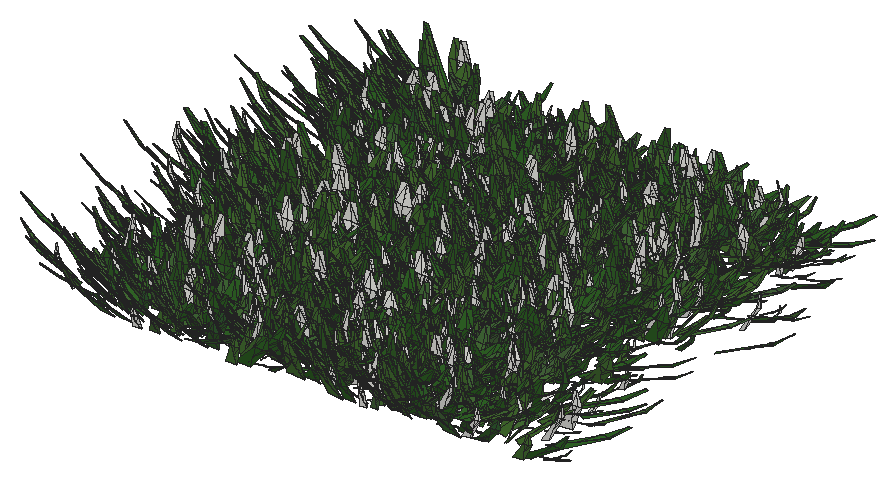
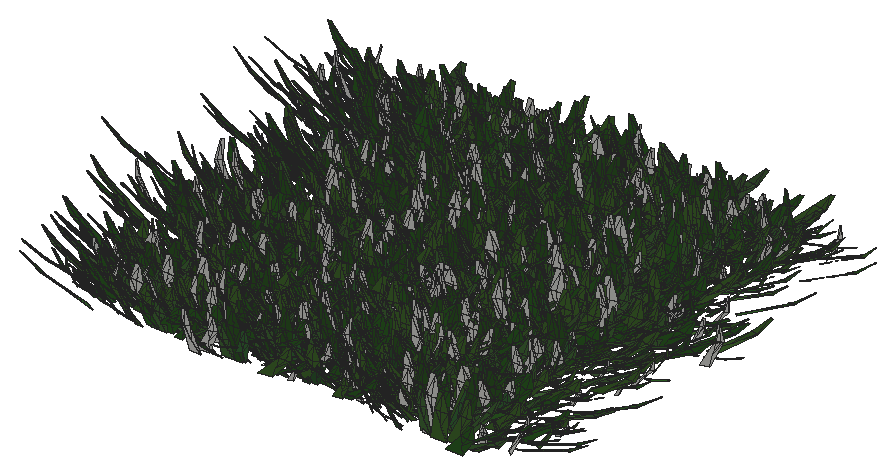
# SketchUp Ruby script. Lengths in inches.
U = 1.inch
M = Sketchup.active_model
def pt(a) = Geom::Point3d.new(a.map { |v| v * U })
def face(e, loops, mat)
  f = e.add_face(loops[0].map { |a| pt(a) })
  loops[1..].each { |l| e.add_face(l.map { |a| pt(a) }).erase! }
  f.material = f.back_material = mat if mat
  f
end
# faces: each face lists its corners as indices into pts; further lists are holes
def faces(e, pts, list, mat = nil) = list.each { |f| face(e, (f[0].is_a?(Array) ? f : [f]).map { |l| l.map { |i| pts[i] } }, mat) }
# xy, xz, yz: faces in a plane at the given z, y or x. An outline is a flat list of corners, or four numbers for a rectangle; further outlines are holes
def ring(l) = l.size == 4 ? [[l[0], l[1]], [l[2], l[1]], [l[2], l[3]], [l[0], l[3]]] : l.each_slice(2).to_a
def flat(e, list, mat, &to3) = list.each { |f| face(e, (f[0].is_a?(Array) ? f : [f]).map { |l| ring(l).map { |u, v| to3.(u, v) } }, mat) }
def xy(e, z, list, mat = nil) = flat(e, list, mat) { |x, y| [x, y, z] }
def xz(e, y, list, mat = nil) = flat(e, list, mat) { |x, z| [x, y, z] }
def yz(e, x, list, mat = nil) = flat(e, list, mat) { |y, z| [x, y, z] }
def lines(e, pts, list) = list.each { |a, b| e.add_line(pt(pts[a]), pt(pts[b])) }
# prism: a flat outline (further loops are holes) pulled along v
def prism(e, loops, v, mat = nil)
  f = face(e, loops, mat); d = Geom::Vector3d.new(v.map { |x| x * U })
  f.pushpull(f.normal.samedirection?(d) ? d.length : -d.length)
end
def box(e, o, s, mat = nil) = prism(e, [[o, [o[0] + s[0], o[1], o[2]], [o[0] + s[0], o[1] + s[1], o[2]], [o[0], o[1] + s[1], o[2]]]], [0, 0, s[2]], mat)
def at(x, y, z, deg = 0) = Geom::Transformation.translation(pt([x, y, z])) * Geom::Transformation.rotation(ORIGIN, Z_AXIS, deg.degrees)
def axes(o, x, y, z) = Geom::Transformation.new([*x, 0, *y, 0, *z, 0, *pt(o).to_a, 1])
def part(name) = M.definitions.add(name)
# library, detail: a bought-in or finely detailed component or shape, given as its bounding box
def library(name, o, s) = part(name).tap { |d| box(d.entities, o, s) }
def detail(e, o, s) = box(e.add_group.entities, o, s)
def put(e, d, t, mat = nil) = e.add_instance(d, t).tap { |i| i.material = mat if mat }
def group(e, t, mat = nil) = e.add_group.tap { |g| g.transformation = t; g.material = mat if mat }.entities
root = M.entities
M.materials.add("Material10").color = [48, 100, 38]
M.materials.add("Material3").color = [68, 110, 58]
M.materials.add("Material4").color = [48, 90, 38]
M.materials.add("Material5").color = [68, 110, 48]
M.materials.add("Material6").color = [48, 90, 48]
M.materials.add("Material7").color = [58, 110, 58]
M.materials.add("Material8").color = [58, 90, 38]
M.materials.add("Material9").color = [68, 100, 58]
c1 = part("grass00")
p = [[-0.6875,0.15,0],[-0.56,0.08,5.52],[-0.04,0.03,2.76],[0.48,-0.02,0],[0.35,-0.02,5.52],[-0.1,-0.14,5.52],
  [-0.12,0.65,8.37],[-0.42,0.65,8.37]]
faces(c1.entities,p,[[0,1,2,3],[3,2,4],[1,5,2],[5,4,2],[1,6,5],[4,5,6],[7,6,1]])
c2 = part("Group16\#1")
put(c2.entities,c1,axes([1.44,-0.61,-0.01],[0.05352,0.12609,0],[-0.10704,0.04543,0.07239],[0.06664,-0.02828,0.11628]),"Material6")
put(c2.entities,c1,axes([0.76,-0.15,-0.01],[0.04676,0.24062,0],[-0.23162,0.04501,0.06642],[0.0652,-0.01267,0.23595]),"Material3")
put(c2.entities,c1,axes([0.79,0.01,-0.01],[-0.00606,0.34651,0],[-0.34381,-0.00602,0.0432],[0.04319,0.00076,0.34386]))
put(c2.entities,c1,axes([1,0.23,-0.01],[-0.07192,0.31144,0],[-0.28722,-0.06632,0.1236],[0.12043,0.02781,0.29478]),"Material5")
put(c2.entities,c1,axes([1.66,0.77,-0.01],[-0.13828,0.29651,0],[-0.21551,-0.1005,0.22471],[0.20365,0.09498,0.23779]),"Material10")
put(c2.entities,c1,axes([0.6875,0.52,-0.01],[-0.18126,0.24051,0],[-0.22746,-0.17142,0.09788],[0.07817,0.05891,0.28481]),"Material5")
put(c2.entities,c1,axes([0.68,0.78,-0.01],[-0.215,0.18688,0],[-0.12385,-0.14248,0.21334],[0.13995,0.16101,0.18878]),"Material3")
put(c2.entities,c1,axes([0.56,1,-0.01],[-0.13756,0.07624,0],[-0.06159,-0.11112,0.0927],[0.04494,0.08108,0.12705]),"Material5")
put(c2.entities,c1,axes([0.2,0.64,-0.01],[-0.23729,0.07254,0],[-0.05711,-0.18681,0.153],[0.04473,0.14632,0.19535]),"Material10")
put(c2.entities,c1,axes([0.0625,0.72,-0.01],[-0.28874,0.02525,0],[-0.02179,-0.24916,0.14647],[0.01276,0.14591,0.25012]),"Material3")
put(c2.entities,c1,axes([-0.08,0.62,-0.01],[-0.34089,-0.04187,0],[0.03255,-0.26504,0.216],[-0.02633,0.21439,0.26703]),"Material10")
put(c2.entities,c1,axes([-0.34,0.98,-0.01],[-0.14314,-0.0493,0],[0.04397,-0.12769,0.06843],[-0.02228,0.0647,0.13505]),"Material10")
put(c2.entities,c1,axes([-0.87,1.45,-0.01],[-0.23488,-0.14114,0],[0.13761,-0.22901,0.06087],[-0.03135,0.05217,0.26717]))
put(c2.entities,c1,axes([-0.72,0.77,-0.01],[-0.14208,-0.13251,0],[0.07209,-0.0773,0.16301],[-0.11118,0.11922,0.1057]),"Material10")
put(c2.entities,c1,axes([-0.62,0.43,-0.01],[-0.14845,-0.21203,0],[0.18654,-0.13061,0.12304],[-0.10079,0.07057,0.22772]),"Material3")
put(c2.entities,c1,axes([-0.68,0.29,-0.01],[-0.13639,-0.32136,0],[0.31723,-0.13464,0.05579],[-0.05136,0.0218,0.34462]),"Material4")
put(c2.entities,c1,axes([-0.64,0.125,-0.01],[-0.0458,-0.23569,0],[0.22124,-0.043,0.08276],[-0.08124,0.01579,0.22538]),"Material7")
put(c2.entities,c1,axes([-1.6,-0.03,-0.01],[0.00576,-0.32897,0],[0.27526,0.00482,0.18018],[-0.18015,-0.00315,0.2753]),"Material5")
put(c2.entities,c1,axes([-1.36,-0.31,-0.01],[0.05718,-0.24765,0],[0.18172,0.04196,0.17267],[-0.16825,-0.03885,0.1865]),"Material10")
put(c2.entities,c1,axes([-1.54,-0.72,-0.01],[0.06537,-0.14017,0],[0.13555,0.06321,0.03939],[-0.0357,-0.01665,0.14956]))
put(c2.entities,c1,axes([-1.19,-0.9,-0.01],[0.09597,-0.12735,0],[0.11214,0.08451,0.07557],[-0.06035,-0.04548,0.14042]),"Material9")
put(c2.entities,c1,axes([-0.47,-0.54,-0.01],[0.11588,-0.10072,0],[0.0618,0.0711,0.12124],[-0.07953,-0.0915,0.0942]))
put(c2.entities,c1,axes([-0.47,-0.84,-0.01],[0.11927,-0.0661,0],[0.06603,0.11913,0.00646],[-0.00313,-0.00565,0.13621]),"Material5")
put(c2.entities,c1,axes([-0.38,-1.24,-0.01],[0.28037,-0.08571,0],[0.0618,0.20215,0.20315],[-0.05939,-0.19428,0.21139]),"Material9")
put(c2.entities,c1,axes([-0.06,-0.66,-0.01],[0.22719,-0.01987,0],[0.01247,0.14255,0.17758],[-0.01547,-0.17691,0.1431]),"Material8")
put(c2.entities,c1,axes([0.11,-0.89,-0.01],[0.14882,0.01828,0],[-0.01058,0.08611,0.12229],[0.01491,-0.12138,0.08676]),"Material6")
put(c2.entities,c1,axes([0.25,-0.72,-0.01],[0.20481,0.07053,0],[-0.06206,0.18022,0.10291],[0.03351,-0.0973,0.1906]),"Material6")
put(c2.entities,c1,axes([0.85,-1.42,-0.01],[0.16481,0.09904,0],[-0.09472,0.15762,0.05616],[0.02893,-0.04814,0.18389]),"Material5")
put(c2.entities,c1,axes([1.01,-1.09,-0.01],[0.21858,0.20385,0],[-0.17495,0.1876,0.15339],[0.10462,-0.11218,0.25652]),"Material10")
put(c2.entities,c1,axes([1.01,-0.71,-0.01],[0.08733,0.12473,0],[-0.06445,0.04512,0.13037],[0.1068,-0.07477,0.07867]),"Material6")
c3 = part("Group15\#1")
put(c3.entities,c2,at(0,0,0))
c4 = part("3darcstudiotree_grass00\#1")
put(c4.entities,c3,at(0,0,0))
put(root,c4,axes([257.86,22.3125,7.6],[3.70549,0.72715,0],[-2.49617,0.79502,-0.02005],[-0.09119,0.02904,1.86077]))
put(root,c4,axes([260.11,41.54,7.6],[0.01218,-1.00906,0],[4.98185,0.00376,-0.03692],[0.18714,0.00014,1.57831]))
put(root,c4,axes([260.48,26.33,7.6],[-1.42025,-0.83489,0],[4.16242,-0.44255,-0.01791],[0.11075,-0.01178,1.89984]))
put(root,c4,axes([260.59,11.3125,7.6],[0.28027,-0.96199,0],[3.64955,0.06646,-0.00937],[0.0792,0.00144,1.93766]))
put(root,c4,axes([260.47,8.13,7.6],[-3.43805,0.34453,0],[-1.648,-1.02783,-0.04281],[-0.10438,-0.0651,1.81418]))
put(root,c4,axes([260.35,37.81,7.6],[3.40925,-0.75567,0],[3.0298,0.85432,-0.03392],[0.10448,0.02946,1.32537]))
put(root,c4,axes([261.56,15.87,7.6],[-4.27926,0.10077,0],[-0.4125,-1.0948,-0.0202],[-0.01348,-0.03577,1.95637]))
put(root,c4,axes([260.31,4.91,7.6],[3.9837,-0.03206,0],[0.11597,0.90077,-0.04101],[0.00803,0.06239,1.37186]))
put(root,c4,axes([260.38,43.39,7.6],[0.14781,1.06815,0],[-4.11052,0.03555,-0.02489],[-0.18669,0.00161,1.9295]))
put(root,c4,axes([261,40.27,7.6],[-2.74206,0.64257,0],[-3.29567,-0.87899,-0.02311],[-0.07278,-0.01941,1.38694]))
put(root,c4,axes([262.26,35.6,7.6],[-4.52462,0.16915,0],[-0.75823,-1.26762,-0.06496],[-0.05656,-0.09455,1.88637]))
put(root,c4,axes([261.375,23.73,7.6],[-1.87065,0.77621,0],[-4.34622,-0.65464,-0.04504],[-0.23728,-0.03574,1.9506]))
put(root,c4,axes([261.58,30.06,7.6],[4.16044,-0.73269,0],[2.40364,0.85303,-0.03692],[0.14968,0.05312,1.83631]))
put(root,c4,axes([261.44,6.63,7.6],[3.59915,0.14594,0],[-0.59052,0.91023,-0.01255],[-0.01426,0.02198,1.63564]))
put(root,c4,axes([262.1,34.35,7.6],[-2.60039,0.90097,0],[-2.99223,-0.53976,-0.00844],[-0.04191,-0.00756,1.41311]))
put(root,c4,axes([261.36,28.15,7.6],[2.59672,0.84047,0],[-3.92214,0.75737,-0.04605],[-0.16947,0.03272,1.44046]))
put(root,c4,axes([262.71,17.81,7.6],[1.82286,-0.79645,0],[3.62821,0.519,-0.04415],[0.29175,0.04173,1.98924]))
put(root,c4,axes([263.91,38.8,7.6],[-0.69021,-1.10068,0],[5.10027,-0.19989,-0.06318],[0.26987,-0.01058,1.39517]))
put(root,c4,axes([262.22,18.82,7.6],[2.76483,1.10064,0],[-3.85856,0.6058,-0.052],[-0.27462,0.04312,1.7759]))
put(root,c4,axes([263.08,33.25,7.6],[3.65122,-0.89135,0],[3.24538,0.83087,-0.04175],[0.1632,0.04178,1.62422]))
put(root,c4,axes([262.42,30.83,7.6],[4.36658,0.08239,0],[-0.38033,1.25977,-0.00004],[-0.00002,0.00006,1.93334]))
put(root,c4,axes([264.22,13.1,7.6],[-2.28283,-1.06843,0],[4.21309,-0.56261,-0.05822],[0.33198,-0.04433,1.92982]))
put(root,c4,axes([263.27,24.83,7.6],[0.26997,1.23611,0],[-4.58463,0.06258,-0.05861],[-0.40129,0.00548,1.96776]))
put(root,c4,axes([262.73,21.11,7.6],[4.48895,0.48675,0],[-1.69756,0.97846,-0.01845],[-0.03711,0.02139,1.34771]))
put(root,c4,axes([262.76,4.1875,7.6],[2.13817,1.11793,0],[-4.20741,0.50295,-0.01048],[-0.04572,0.00547,1.40926]))
put(root,c4,axes([263.12,14.4375,7.6],[4.31033,0.25907,0],[-1.20979,1.25799,-0.03506],[-0.03358,0.03491,1.32515]))
put(root,c4,axes([263.83,10.03,7.6],[4.12313,-0.24157,0],[1.18082,1.25966,-0.02268],[0.02474,0.0264,1.5468]))
put(root,c4,axes([263.82,21.84,7.6],[-0.03316,1.25701,0],[-4.94993,-0.00816,-0.01347],[-0.06338,-0.0001,1.45625]))
put(root,c4,axes([266.25,8.97,7.6],[3.15531,-0.58243,0],[2.70786,0.91686,-0.02283],[0.06907,0.02339,1.4512]))
put(root,c4,axes([267.25,12.4375,7.6],[-1.85827,-1.20054,0],[4.6379,-0.44867,-0.05475],[0.3098,-0.02997,1.88574]))
put(root,c4,axes([266.25,6.97,7.6],[3.52758,-0.61527,0],[2.26758,0.81256,-0.00731],[0.03042,0.0109,1.80073]))
put(root,c4,axes([267.49,41.7,7.6],[-2.08937,-0.99009,0],[3.80908,-0.50239,-0.03938],[0.17969,-0.0237,1.38871]))
put(root,c4,axes([266.46,32.39,7.6],[3.90144,-0.65649,0],[2.04826,0.76078,-0.0013],[0.00472,0.00175,1.49257]))
put(root,c4,axes([266.35,14.87,7.6],[-1.15605,0.94536,0],[-4.28561,-0.32755,-0.0271],[-0.16007,-0.01223,1.72974]))
put(root,c4,axes([267.77,9.78,7.6],[-4.45544,0.35262,0],[-1.28974,-1.0185,-0.03323],[-0.0666,-0.05259,1.77353]))
put(root,c4,axes([266.74,5.17,7.6],[4.66445,0.12304,0],[-0.40469,0.95886,-0.03171],[-0.02368,0.05611,1.71518]))
put(root,c4,axes([268.5,16.46,7.6],[0.22891,-1.1855,0],[4.26581,0.05148,-0.00402],[0.01994,0.00024,1.3243]))
put(root,c4,axes([268.62,20.7,7.6],[-3.83276,-0.4307,0],[1.47756,-0.82179,-0.02079],[0.061,-0.03393,1.61237]))
put(root,c4,axes([267.81,22.21,7.6],[-2.46367,0.88426,0],[-3.17691,-0.55321,-0.01437],[-0.09353,-0.01629,1.91898]))
put(root,c4,axes([268.79,37.76,7.6],[-2.3426,-0.88357,0],[3.5724,-0.59197,-0.05028],[0.30493,-0.05053,1.94898]))
put(root,c4,axes([267.56,40.5,7.6],[4.40447,-0.22368,0],[0.75254,0.92613,-0.00331],[0.00443,0.00545,1.58887]))
put(root,c4,axes([267,31,7.6],[4.73855,0.38676,0],[-1.49783,1.14695,-0.00124],[-0.0021,0.00161,1.65228]))
put(root,c4,axes([268.3125,36.125,7.6],[-1.79093,0.80578,0],[-3.73339,-0.51862,-0.05151],[-0.32129,-0.04463,1.90487]))
put(root,c4,axes([267.44,34.1,7.6],[1.1144,0.95521,0],[-4.67069,0.34057,-0.00405],[-0.01733,0.00126,1.35389]))
put(root,c4,axes([269.95,28.47,7.6],[-3.69018,-0.70839,0],[2.67455,-0.87078,-0.00705],[0.02875,-0.00936,1.8369]))
put(root,c4,axes([269.01,29.5625,7.6],[2.21238,-0.82212,0],[4.12079,0.69308,-0.06298],[0.2244,0.03774,1.33293]))
put(root,c4,axes([268.15,4.13,7.6],[4.71925,-0.11324,0],[0.46781,1.21853,-0.01064],[0.0059,0.01536,1.77558]))
put(root,c4,axes([270.09,39.03,7.6],[-3.23059,-0.98889,0],[3.90689,-0.79771,-0.03335],[0.15229,-0.03109,1.85855]))
put(root,c4,axes([269.45,25.67,7.6],[0.38736,-1.28995,0],[5.0857,0.09545,-0.06273],[0.38626,0.00725,1.9684]))
put(root,c4,axes([269.01,11.0625,7.6],[-1.91482,0.78597,0],[-3.52393,-0.53658,-0.03041],[-0.133,-0.02025,1.3205]))
put(root,c4,axes([270.46,24.12,7.6],[-1.97779,-0.85605,0],[3.47193,-0.50134,-0.00817],[0.04391,-0.00634,1.55447]))
put(root,c4,axes([269.63,26.14,7.6],[4.07935,-0.43346,0],[1.89845,1.11667,-0.00549],[0.0102,0.006,1.44062]))
put(root,c4,axes([269.625,17.95,7.6],[4.37754,-0.30034,0],[1.33809,1.21894,-0.05143],[0.06212,0.05659,1.44218]))
put(root,c4,axes([269.58,19.21,7.6],[-0.77459,1.02893,0],[-4.84534,-0.22797,-0.01956],[-0.11313,-0.00532,1.8138]))
put(root,c4,axes([272.3,16.35,7.6],[-4.74279,0.28772,0],[-1.21823,-1.25511,-0.06662],[-0.06794,-0.07,1.39642]))
put(root,c4,axes([273.27,9.5,7.6],[-3.58073,-0.35661,0],[1.83074,-1.1489,-0.00121],[0.00279,-0.00175,1.92636]))
put(root,c4,axes([272.43,40.28,7.6],[1.54312,-0.81512,0],[3.29472,0.38983,-0.04441],[0.34585,0.04092,1.96303]))
put(root,c4,axes([273.24,37.31,7.6],[-0.36487,-0.9693,0],[3.80087,-0.08942,-0.04952],[0.26852,-0.00632,1.29958]))
put(root,c4,axes([273.36,34.29,7.6],[-3.87388,0.80913,0],[-2.80413,-0.83909,-0.03098],[-0.11588,-0.03468,1.59479]))
put(root,c4,axes([274.03,42.92,7.6],[-4.21097,-0.15572,0],[0.54772,-0.92572,-0.00812],[0.00706,-0.01193,1.3892]))
put(root,c4,axes([273.51,30.9,7.6],[-3.28993,0.53414,0],[-2.35898,-0.90811,-0.04277],[-0.16039,-0.06174,1.86401]))
put(root,c4,axes([272.92,11.22,7.6],[-0.64164,1.09647,0],[-3.76994,-0.13788,-0.02144],[-0.17386,-0.00636,1.9513]))
put(root,c4,axes([273.48,25.67,7.6],[-3.33719,0.61695,0],[-2.63683,-0.89144,-0.01371],[-0.03862,-0.01306,1.31321]))
put(root,c4,axes([272.92,39.17,7.6],[3.65959,-0.0096,0],[0.04442,1.05836,-0.01029],[0.00057,0.0135,1.389]))
put(root,c4,axes([274.16,14.41,7.6],[1.63627,-0.81784,0],[3.89049,0.48648,-0.01805],[0.09406,0.01176,1.58457]))
put(root,c4,axes([273.19,29.82,7.6],[4.2926,-0.51485,0],[1.76165,0.91799,-0.04597],[0.12323,0.06421,1.57738]))
put(root,c4,axes([273.39,27.92,7.6],[-2.40518,0.923,0],[-4.34744,-0.70804,-0.00953],[-0.03635,-0.00592,1.47621]))
put(root,c4,axes([274.76,41.96,7.6],[1.06062,-0.94983,0],[4.26034,0.29733,-0.00232],[0.01421,0.00099,1.76107]))
put(root,c4,axes([273.67,32.91,7.6],[3.58152,-0.18688,0],[0.799,0.95704,-0.04941],[0.06002,0.07189,1.4533]))
put(root,c4,axes([275.01,21.13,7.6],[2.30537,-0.84658,0],[3.6231,0.61664,-0.01892],[0.09951,0.01694,1.74337]))
put(root,c4,axes([274.88,6.4375,7.6],[-2.37312,0.89049,0],[-3.32471,-0.55376,-0.03773],[-0.17795,-0.02964,1.41517]))
put(root,c4,axes([274.04,35.61,7.6],[4.42223,0.30333,0],[-1.18434,1.07915,-0.02738],[-0.04878,0.04444,1.88342]))
put(root,c4,axes([274.64,26.125,7.6],[4.7526,-0.49648,0],[1.99217,1.19189,-0.05614],[0.10535,0.06303,1.57175]))
put(root,c4,axes([275.75,18.03,7.6],[2.12632,-1.16665,0],[4.03974,0.46017,-0.02827],[0.17992,0.0205,1.94019]))
put(root,c4,axes([274.99,22.12,7.6],[0.82616,1.18847,0],[-3.57688,0.1554,-0.03272],[-0.26216,0.01139,1.8454]))
put(root,c4,axes([274.7,23.68,7.6],[3.22998,0.67416,0],[-3.0562,0.91516,-0.05497],[-0.20916,0.06263,1.76958]))
put(root,c4,axes([274.67,18.53,7.6],[2.39946,0.73907,0],[-3.00526,0.6098,-0.00448],[-0.02213,0.00449,1.5389]))
put(root,c4,axes([275.9375,13.2,7.6],[2.55238,-0.83938,0],[4.10588,0.78031,-0.05929],[0.21983,0.04178,1.50135]))
put(root,c4,axes([275.66,5.375,7.6],[-0.55541,1.00886,0],[-4.55532,-0.15674,-0.0385],[-0.20653,-0.00711,1.55608]))
put(root,c4,axes([276.09,8.625,7.6],[4.68045,-0.41888,0],[1.5867,1.1081,-0.05713],[0.0969,0.06767,1.48067]))
put(root,c4,axes([278.32,35.37,7.6],[-3.20384,-1.02326,0],[3.97726,-0.7783,-0.01534],[0.06587,-0.01289,1.72134]))
put(root,c4,axes([278.09,25.28,7.6],[-4.59803,0.08563,0],[-0.2847,-0.9555,-0.0204],[-0.00865,-0.02903,1.3669]))
put(root,c4,axes([278.49,38.61,7.6],[-4.38136,-0.40254,0],[1.40005,-0.95241,-0.00277],[0.00519,-0.00353,1.38049]))
put(root,c4,axes([279.07,27,7.6],[-3.71243,-0.56774,0],[2.64786,-1.08214,-0.03935],[0.09328,-0.03812,1.44076]))
put(root,c4,axes([278.32,8.16,7.6],[4.21231,-0.52689,0],[1.66569,0.83229,-0.01525],[0.04687,0.02342,1.59832]))
put(root,c4,axes([279.01,31.22,7.6],[2.41687,-0.67519,0],[3.02095,0.67585,-0.01984],[0.10631,0.02378,1.82222]))
put(root,c4,axes([278.8125,27.77,7.6],[0.7487,1.19338,0],[-3.70978,0.14547,-0.03929],[-0.32325,0.01268,1.95437]))
put(root,c4,axes([280.43,32.6875,7.6],[-2.24094,-0.73195,0],[3.39914,-0.65043,-0.02737],[0.10576,-0.02024,1.30175]))
put(root,c4,axes([279.25,23.34,7.6],[-0.31652,1.20504,0],[-3.66531,-0.06017,-0.03425],[-0.24045,-0.00395,1.61497]))
put(root,c4,axes([280.17,37.56,7.6],[1.87547,-0.90536,0],[3.87003,0.50105,-0.01075],[0.05218,0.00676,1.48923]))
put(root,c4,axes([280.47,14.07,7.6],[-4.13074,0.02619,0],[-0.11371,-1.1209,-0.00196],[-0.00027,-0.00262,1.49745]))
put(root,c4,axes([279.75,10.17,7.6],[-2.5882,0.79848,0],[-3.68123,-0.74577,-0.04128],[-0.16563,-0.03355,1.52936]))
put(root,c4,axes([279.28,13.23,7.6],[4.43719,0.0399,0],[-0.16058,1.11619,-0.02702],[-0.00694,0.04824,1.99535]))
put(root,c4,axes([280.27,43.73,7.6],[2.51749,-0.66921,0],[3.09976,0.7288,-0.02136],[0.09486,0.0223,1.62144]))
put(root,c4,axes([281.07,11.69,7.6],[-4.57103,-0.1339,0],[0.44169,-0.94237,-0.00847],[0.00759,-0.0162,1.82708]))
put(root,c4,axes([279.92,30.03,7.6],[1.81154,0.83974,0],[-3.36309,0.45344,-0.03445],[-0.23344,0.03147,1.83855]))
put(root,c4,axes([281.78,7.5,7.6],[-3.18482,-0.5306,0],[2.64212,-0.99117,-0.04785],[0.16263,-0.06101,1.82518]))
put(root,c4,axes([280.72,21.1,7.6],[-1.1436,1.00471,0],[-3.56675,-0.25374,-0.00052],[-0.00362,-0.00026,1.67384]))
put(root,c4,axes([280.86,21.85,7.6],[4.19446,0.12436,0],[-0.54634,1.15167,-0.05841],[-0.03094,0.06521,1.30397]))
put(root,c4,axes([282.52,17.11,7.6],[-3.94605,-0.19743,0],[0.76142,-0.95114,-0.00178],[0.00253,-0.00316,1.75352]))
put(root,c4,axes([281.92,34.03,7.6],[-3.21823,0.62251,0],[-2.5621,-0.82785,-0.04163],[-0.13582,-0.04388,1.39503]))
put(root,c4,axes([280.98,40.03,7.6],[2.86514,0.59771,0],[-2.37877,0.71266,-0.00812],[-0.03621,0.01085,1.6158]))
put(root,c4,axes([280.9375,16.24,7.6],[2.40396,0.87072,0],[-3.51835,0.60711,-0.02215],[-0.11639,0.02008,1.70619]))
put(root,c4,axes([281.67,4.88,7.6],[0.47461,1.07377,0],[-3.68217,0.10172,-0.03685],[-0.27492,0.00759,1.73767]))
put(root,c4,axes([281.27,41.3,7.6],[4.18661,0.73977,0],[-2.83874,1.00409,-0.0169],[-0.04607,0.01629,1.45184]))
put(root,c4,axes([282.3,19.04,7.6],[4.09522,-0.17448,0],[0.64394,0.9446,-0.03176],[0.04135,0.06066,1.85682]))
put(root,c4,axes([284.35,14.17,7.6],[-2.585,-1.04322,0],[3.07878,-0.47681,-0.00146],[0.00727,-0.00113,1.32424]))
put(root,c4,axes([284.3,10.35,7.6],[4.12343,-0.57612,0],[2.31328,1.0348,-0.04605],[0.10519,0.04706,1.38783]))
put(root,c4,axes([285.6875,8.24,7.6],[-3.01934,-0.67461,0],[2.59527,-0.72597,-0.04195],[0.17887,-0.05004,1.55746]))
put(root,c4,axes([284.12,40.2,7.6],[1.24737,1.15044,0],[-4.46094,0.3023,-0.03421],[-0.2215,0.01501,1.93796]))
put(root,c4,axes([286.31,19.53,7.6],[-1.14351,-1.16914,0],[4.8405,-0.2959,-0.03172],[0.13527,-0.00827,1.36741]))
put(root,c4,axes([286.48,5.45,7.6],[-3.21504,-0.48766,0],[2.28718,-0.94243,-0.00574],[0.01454,-0.00599,1.3472]))
put(root,c4,axes([286.51,25.63,7.6],[-3.15035,-0.75707,0],[2.9131,-0.75763,-0.02949],[0.15297,-0.03979,1.96656]))
put(root,c4,axes([286.66,29.42,7.6],[-3.24274,-0.9643,0],[3.00099,-0.63073,-0.02964],[0.15134,-0.03181,1.63454]))
put(root,c4,axes([284.92,17.9,7.6],[3.01617,0.89347,0],[-2.94209,0.62075,-0.05003],[-0.28997,0.06118,1.82479]))
put(root,c4,axes([285.1,22.2,7.6],[2.5933,0.94523,0],[-3.23927,0.55545,-0.03781],[-0.2219,0.03805,1.74723]))
put(root,c4,axes([285.16,41.79,7.6],[4.89603,0.07684,0],[-0.28824,1.14785,-0.04601],[-0.01316,0.0524,1.31249]))
put(root,c4,axes([285.87,28.27,7.6],[-2.72717,0.91933,0],[-3.49968,-0.64886,-0.0152],[-0.05921,-0.01098,1.3203]))
put(root,c4,axes([285.26,23.07,7.6],[1.14482,1.02843,0],[-4.70727,0.3275,-0.02844],[-0.16339,0.01137,1.82107]))
put(root,c4,axes([286.11,37.31,7.6],[-2.54341,1.08635,0],[-4.03419,-0.59031,-0.03733],[-0.16382,-0.02397,1.48568]))
put(root,c4,axes([285.44,33.74,7.6],[2.27146,0.75873,0],[-3.43794,0.64327,-0.0157],[-0.07531,0.01409,1.60759]))
put(root,c4,axes([286.21,20.16,7.6],[3.97684,-0.65785,0],[2.37523,0.89742,-0.03005],[0.11618,0.04389,1.88475]))
put(root,c4,axes([285.76,27.18,7.6],[0.9962,1.21765,0],[-4.18163,0.21382,-0.01369],[-0.07051,0.00361,1.40267]))
put(root,c4,axes([286.41,6.99,7.6],[0.30444,1.1436,0],[-4.22382,0.07028,-0.01024],[-0.07034,0.00117,1.82096]))
put(root,c4,axes([286.96,32.16,7.6],[-1.34742,1.17452,0],[-4.20278,-0.30134,-0.02925],[-0.13999,-0.01004,1.36051]))
put(root,c4,axes([286.59,36.05,7.6],[2.73951,0.74881,0],[-3.24608,0.74223,-0.03451],[-0.17558,0.04015,1.89576]))
put(root,c4,axes([286.75,39.09,7.6],[4.21944,0.50022,0],[-1.55878,0.82178,-0.0026],[-0.00889,0.00468,1.81639]))
put(root,c4,axes([288.46,13.0625,7.6],[-4.32099,0.14556,0],[-0.59248,-1.09927,-0.01091],[-0.0098,-0.01818,1.8656]))
put(root,c4,axes([286.97,10.96,7.6],[5.12297,0.07434,0],[-0.27761,1.19572,-0.0212],[-0.00806,0.03474,1.96575]))
put(root,c4,axes([287.29,30.93,7.6],[4.26894,0.36032,0],[-1.62732,1.205,-0.0473],[-0.09046,0.06698,1.90097]))
put(root,c4,axes([287.36,43.63,7.6],[4.07758,0.30015,0],[-1.15535,0.98096,-0.01058],[-0.01796,0.01525,1.53588]))
put(root,c4,axes([287.54,16,7.6],[3.97096,0.2686,0],[-1.03044,0.95214,-0.04799],[-0.08149,0.0753,1.60328]))
put(root,c4,axes([290.93,8.64,7.6],[-3.00965,-0.629,0],[2.74401,-0.82061,-0.04185],[0.17493,-0.05231,1.7425]))
put(root,c4,axes([291.23,30.875,7.6],[-2.42345,-0.78583,0],[3.59047,-0.69205,-0.03514],[0.17335,-0.03341,1.76492]))
put(root,c4,axes([291.16,38.74,7.6],[1.70921,-0.84435,0],[3.84914,0.48698,-0.00728],[0.03207,0.00406,1.33141]))
put(root,c4,axes([290.6,40.22,7.6],[-1.51485,1.06951,0],[-3.50861,-0.3106,-0.04758],[-0.30375,-0.02689,1.57537]))
put(root,c4,axes([291.75,11.53,7.6],[-4.50974,-0.37005,0],[1.35893,-1.03507,-0.0393],[0.07695,-0.05861,1.71017]))
put(root,c4,axes([291.28,33.05,7.6],[-4.37049,0.5936,0],[-1.84843,-0.85059,-0.00649],[-0.01819,-0.00837,1.42064]))
put(root,c4,axes([290.57,41.97,7.6],[-0.14514,1.16082,0],[-3.94632,-0.03084,-0.04056],[-0.22687,-0.00177,1.38085]))
put(root,c4,axes([291.5,18.52,7.6],[-2.03317,0.85161,0],[-3.54583,-0.52909,-0.0186],[-0.09087,-0.01356,1.46845]))
put(root,c4,axes([291.7,26.09,7.6],[3.9809,-0.25729,0],[1.14083,1.10321,-0.04398],[0.07296,0.07055,1.88821]))
put(root,c4,axes([291.64,5.66,7.6],[4.79923,0.3708,0],[-1.47799,1.19558,-0.04987],[-0.07603,0.0615,1.61513]))
